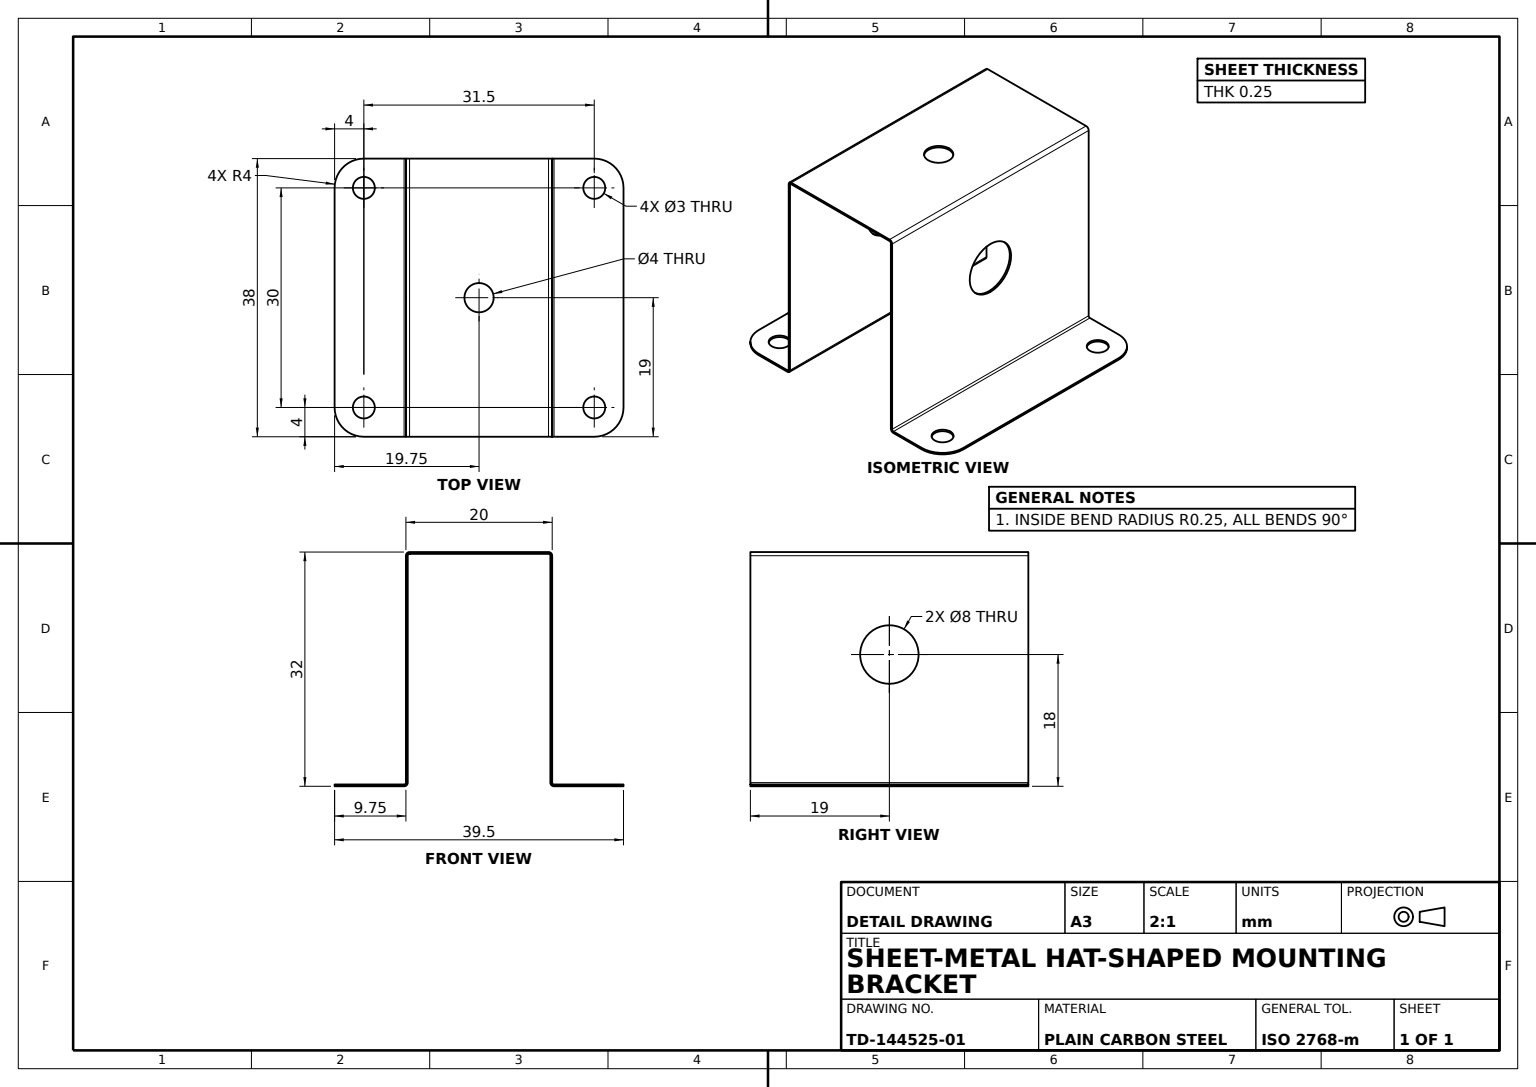
ISO-10303-21;
HEADER;
FILE_DESCRIPTION((''),'2;1');
FILE_NAME('','',(''),(''),'','','');
FILE_SCHEMA(('AUTOMOTIVE_DESIGN'));
ENDSEC;
DATA;
#1=APPLICATION_CONTEXT('');
#2=PRODUCT_CONTEXT('',#1,'mechanical');
#3=PRODUCT('','','',(#2));
#4=PRODUCT_DEFINITION_FORMATION('','',#3);
#5=PRODUCT_DEFINITION_CONTEXT('',#1,'design');
#6=PRODUCT_DEFINITION('','',#4,#5);
#7=PRODUCT_DEFINITION_SHAPE('','',#6);
#8=(LENGTH_UNIT()NAMED_UNIT(*)SI_UNIT(.MILLI.,.METRE.));
#9=(NAMED_UNIT(*)PLANE_ANGLE_UNIT()SI_UNIT($,.RADIAN.));
#10=(NAMED_UNIT(*)SI_UNIT($,.STERADIAN.)SOLID_ANGLE_UNIT());
#11=UNCERTAINTY_MEASURE_WITH_UNIT(LENGTH_MEASURE(1.E-05),#8,'distance_accuracy_value','');
#12=(GEOMETRIC_REPRESENTATION_CONTEXT(3)GLOBAL_UNCERTAINTY_ASSIGNED_CONTEXT((#11))GLOBAL_UNIT_ASSIGNED_CONTEXT((#8,#9,#10))REPRESENTATION_CONTEXT('',''));
#13=CARTESIAN_POINT('',(-10.25,-31.75,-19.));
#14=VERTEX_POINT('',#13);
#15=CARTESIAN_POINT('',(-10.25,-32.,-19.));
#16=VERTEX_POINT('',#15);
#17=DIRECTION('',(0.,-1.,0.));
#18=VECTOR('',#17,1000.);
#19=LINE('',#15,#18);
#20=EDGE_CURVE('',#14,#16,#19,.T.);
#21=ORIENTED_EDGE('',*,*,#20,.T.);
#22=CARTESIAN_POINT('',(-15.75,-32.,-19.));
#23=VERTEX_POINT('',#22);
#24=CARTESIAN_POINT('',(0.,-32.,-19.));
#25=DIRECTION('',(1.,0.,0.));
#26=VECTOR('',#25,1000.);
#27=LINE('',#24,#26);
#28=EDGE_CURVE('',#23,#16,#27,.T.);
#29=ORIENTED_EDGE('',*,*,#28,.F.);
#30=CARTESIAN_POINT('',(-15.75,-31.75,-19.));
#31=VERTEX_POINT('',#30);
#32=DIRECTION('',(0.,1.,0.));
#33=VECTOR('',#32,1000.);
#34=LINE('',#22,#33);
#35=EDGE_CURVE('',#23,#31,#34,.T.);
#36=ORIENTED_EDGE('',*,*,#35,.T.);
#37=CARTESIAN_POINT('',(-10.,-31.75,-19.));
#38=LINE('',#37,#26);
#39=EDGE_CURVE('',#31,#14,#38,.T.);
#40=ORIENTED_EDGE('',*,*,#39,.T.);
#41=EDGE_LOOP('',(#21,#29,#36,#40));
#42=FACE_OUTER_BOUND('',#41,.T.);
#43=CARTESIAN_POINT('',(-10.,-32.,-19.));
#44=DIRECTION('',(0.,0.,1.));
#45=AXIS2_PLACEMENT_3D('',#43,#44,#25);
#46=PLANE('',#45);
#47=ADVANCED_FACE('',(#42),#46,.F.);
#48=CARTESIAN_POINT('',(9.75,-0.5,19.));
#49=VERTEX_POINT('',#48);
#50=CARTESIAN_POINT('',(9.5,-0.25,19.));
#51=VERTEX_POINT('',#50);
#52=CARTESIAN_POINT('',(9.5,-0.5,19.));
#53=AXIS2_PLACEMENT_3D('',#52,#44,#25);
#54=CIRCLE('',#53,0.25);
#55=EDGE_CURVE('',#49,#51,#54,.T.);
#56=ORIENTED_EDGE('',*,*,#55,.T.);
#57=CARTESIAN_POINT('',(9.5,-0.25,-19.));
#58=VERTEX_POINT('',#57);
#59=DIRECTION('',(0.,0.,-1.));
#60=VECTOR('',#59,1000.);
#61=LINE('',#50,#60);
#62=EDGE_CURVE('',#51,#58,#61,.T.);
#63=ORIENTED_EDGE('',*,*,#62,.T.);
#64=CARTESIAN_POINT('',(9.75,-0.5,-19.));
#65=VERTEX_POINT('',#64);
#66=CARTESIAN_POINT('',(9.5,-0.5,-19.));
#67=DIRECTION('',(-1.,0.,0.));
#68=AXIS2_PLACEMENT_3D('',#66,#59,#67);
#69=CIRCLE('',#68,0.25);
#70=EDGE_CURVE('',#58,#65,#69,.T.);
#71=ORIENTED_EDGE('',*,*,#70,.T.);
#72=VECTOR('',#44,1000.);
#73=LINE('',#64,#72);
#74=EDGE_CURVE('',#65,#49,#73,.T.);
#75=ORIENTED_EDGE('',*,*,#74,.T.);
#76=EDGE_LOOP('',(#56,#63,#71,#75));
#77=FACE_OUTER_BOUND('',#76,.T.);
#78=CARTESIAN_POINT('',(9.5,-0.5,-38.005387));
#79=AXIS2_PLACEMENT_3D('',#78,#44,#25);
#80=CYLINDRICAL_SURFACE('',#79,0.25);
#81=ADVANCED_FACE('',(#77),#80,.F.);
#82=CARTESIAN_POINT('',(-9.5,-0.25,19.));
#83=VERTEX_POINT('',#82);
#84=CARTESIAN_POINT('',(-9.75,-0.5,19.));
#85=VERTEX_POINT('',#84);
#86=CARTESIAN_POINT('',(-9.5,-0.5,19.));
#87=AXIS2_PLACEMENT_3D('',#86,#44,#25);
#88=CIRCLE('',#87,0.25);
#89=EDGE_CURVE('',#83,#85,#88,.T.);
#90=ORIENTED_EDGE('',*,*,#89,.F.);
#91=CARTESIAN_POINT('',(-9.5,0.,19.));
#92=VERTEX_POINT('',#91);
#93=LINE('',#82,#33);
#94=EDGE_CURVE('',#83,#92,#93,.T.);
#95=ORIENTED_EDGE('',*,*,#94,.T.);
#96=CARTESIAN_POINT('',(-10.,-0.5,19.));
#97=VERTEX_POINT('',#96);
#98=AXIS2_PLACEMENT_3D('',#86,#44,#67);
#99=CIRCLE('',#98,0.5);
#100=EDGE_CURVE('',#92,#97,#99,.T.);
#101=ORIENTED_EDGE('',*,*,#100,.T.);
#102=VECTOR('',#67,1000.);
#103=LINE('',#96,#102);
#104=EDGE_CURVE('',#85,#97,#103,.T.);
#105=ORIENTED_EDGE('',*,*,#104,.F.);
#106=EDGE_LOOP('',(#90,#95,#101,#105));
#107=FACE_OUTER_BOUND('',#106,.T.);
#108=AXIS2_PLACEMENT_3D('',#86,#59,#67);
#109=PLANE('',#108);
#110=ADVANCED_FACE('',(#107),#109,.F.);
#111=CARTESIAN_POINT('',(-9.75,-18.,0.));
#112=VERTEX_POINT('',#111);
#113=CARTESIAN_POINT('',(-9.75,-10.,0.));
#114=VERTEX_POINT('',#113);
#115=CARTESIAN_POINT('',(-9.75,-14.,0.));
#116=AXIS2_PLACEMENT_3D('',#115,#67,#17);
#117=CIRCLE('',#116,4.);
#118=EDGE_CURVE('',#112,#114,#117,.T.);
#119=ORIENTED_EDGE('',*,*,#118,.F.);
#120=CARTESIAN_POINT('',(-10.,-18.,0.));
#121=VERTEX_POINT('',#120);
#122=CARTESIAN_POINT('',(19.75,-18.,0.));
#123=LINE('',#122,#102);
#124=EDGE_CURVE('',#112,#121,#123,.T.);
#125=ORIENTED_EDGE('',*,*,#124,.T.);
#126=CARTESIAN_POINT('',(-10.,-10.,0.));
#127=VERTEX_POINT('',#126);
#128=CARTESIAN_POINT('',(-10.,-14.,0.));
#129=AXIS2_PLACEMENT_3D('',#128,#67,#17);
#130=CIRCLE('',#129,4.);
#131=EDGE_CURVE('',#121,#127,#130,.T.);
#132=ORIENTED_EDGE('',*,*,#131,.T.);
#133=CARTESIAN_POINT('',(19.75,-10.,0.));
#134=LINE('',#133,#102);
#135=EDGE_CURVE('',#114,#127,#134,.T.);
#136=ORIENTED_EDGE('',*,*,#135,.F.);
#137=EDGE_LOOP('',(#119,#125,#132,#136));
#138=FACE_OUTER_BOUND('',#137,.T.);
#139=CARTESIAN_POINT('',(19.75,-14.,0.));
#140=AXIS2_PLACEMENT_3D('',#139,#67,#17);
#141=CYLINDRICAL_SURFACE('',#140,4.);
#142=ADVANCED_FACE('',(#138),#141,.F.);
#143=CARTESIAN_POINT('',(10.,-10.,0.));
#144=VERTEX_POINT('',#143);
#145=CARTESIAN_POINT('',(10.,-18.,0.));
#146=VERTEX_POINT('',#145);
#147=CARTESIAN_POINT('',(10.,-14.,0.));
#148=AXIS2_PLACEMENT_3D('',#147,#25,#32);
#149=CIRCLE('',#148,4.);
#150=EDGE_CURVE('',#144,#146,#149,.T.);
#151=ORIENTED_EDGE('',*,*,#150,.T.);
#152=CARTESIAN_POINT('',(9.75,-18.,0.));
#153=VERTEX_POINT('',#152);
#154=EDGE_CURVE('',#146,#153,#123,.T.);
#155=ORIENTED_EDGE('',*,*,#154,.T.);
#156=CARTESIAN_POINT('',(9.75,-10.,0.));
#157=VERTEX_POINT('',#156);
#158=CARTESIAN_POINT('',(9.75,-14.,0.));
#159=AXIS2_PLACEMENT_3D('',#158,#25,#32);
#160=CIRCLE('',#159,4.);
#161=EDGE_CURVE('',#157,#153,#160,.T.);
#162=ORIENTED_EDGE('',*,*,#161,.F.);
#163=EDGE_CURVE('',#144,#157,#134,.T.);
#164=ORIENTED_EDGE('',*,*,#163,.F.);
#165=EDGE_LOOP('',(#151,#155,#162,#164));
#166=FACE_OUTER_BOUND('',#165,.T.);
#167=ADVANCED_FACE('',(#166),#141,.F.);
#168=CARTESIAN_POINT('',(-9.75,-0.5,-19.));
#169=VERTEX_POINT('',#168);
#170=CARTESIAN_POINT('',(-10.,-0.5,-19.));
#171=VERTEX_POINT('',#170);
#172=LINE('',#168,#102);
#173=EDGE_CURVE('',#169,#171,#172,.T.);
#174=ORIENTED_EDGE('',*,*,#173,.T.);
#175=CARTESIAN_POINT('',(-9.5,0.,-19.));
#176=VERTEX_POINT('',#175);
#177=CARTESIAN_POINT('',(-9.5,-0.5,-19.));
#178=AXIS2_PLACEMENT_3D('',#177,#59,#67);
#179=CIRCLE('',#178,0.5);
#180=EDGE_CURVE('',#171,#176,#179,.T.);
#181=ORIENTED_EDGE('',*,*,#180,.T.);
#182=CARTESIAN_POINT('',(-9.5,-0.25,-19.));
#183=VERTEX_POINT('',#182);
#184=LINE('',#182,#33);
#185=EDGE_CURVE('',#183,#176,#184,.T.);
#186=ORIENTED_EDGE('',*,*,#185,.F.);
#187=CIRCLE('',#178,0.25);
#188=EDGE_CURVE('',#169,#183,#187,.T.);
#189=ORIENTED_EDGE('',*,*,#188,.F.);
#190=EDGE_LOOP('',(#174,#181,#186,#189));
#191=FACE_OUTER_BOUND('',#190,.T.);
#192=AXIS2_PLACEMENT_3D('',#177,#44,#25);
#193=PLANE('',#192);
#194=ADVANCED_FACE('',(#191),#193,.F.);
#195=CARTESIAN_POINT('',(-15.75,-31.75,19.));
#196=VERTEX_POINT('',#195);
#197=CARTESIAN_POINT('',(-15.75,-32.,19.));
#198=VERTEX_POINT('',#197);
#199=LINE('',#197,#18);
#200=EDGE_CURVE('',#196,#198,#199,.T.);
#201=ORIENTED_EDGE('',*,*,#200,.F.);
#202=CARTESIAN_POINT('',(-19.75,-31.75,15.));
#203=VERTEX_POINT('',#202);
#204=CARTESIAN_POINT('',(-15.75,-31.75,15.));
#205=AXIS2_PLACEMENT_3D('',#204,#32,#44);
#206=CIRCLE('',#205,4.);
#207=EDGE_CURVE('',#203,#196,#206,.T.);
#208=ORIENTED_EDGE('',*,*,#207,.F.);
#209=CARTESIAN_POINT('',(-19.75,-32.,15.));
#210=VERTEX_POINT('',#209);
#211=LINE('',#209,#33);
#212=EDGE_CURVE('',#210,#203,#211,.T.);
#213=ORIENTED_EDGE('',*,*,#212,.F.);
#214=CARTESIAN_POINT('',(-15.75,-32.,15.));
#215=AXIS2_PLACEMENT_3D('',#214,#17,#44);
#216=CIRCLE('',#215,4.);
#217=EDGE_CURVE('',#198,#210,#216,.T.);
#218=ORIENTED_EDGE('',*,*,#217,.F.);
#219=EDGE_LOOP('',(#201,#208,#213,#218));
#220=FACE_OUTER_BOUND('',#219,.T.);
#221=AXIS2_PLACEMENT_3D('',#214,#32,#67);
#222=CYLINDRICAL_SURFACE('',#221,4.);
#223=ADVANCED_FACE('',(#220),#222,.T.);
#224=CARTESIAN_POINT('',(10.25,-32.,-19.));
#225=VERTEX_POINT('',#224);
#226=CARTESIAN_POINT('',(15.75,-32.,-19.));
#227=VERTEX_POINT('',#226);
#228=EDGE_CURVE('',#225,#227,#27,.T.);
#229=ORIENTED_EDGE('',*,*,#228,.F.);
#230=CARTESIAN_POINT('',(10.25,-31.75,-19.));
#231=VERTEX_POINT('',#230);
#232=LINE('',#230,#18);
#233=EDGE_CURVE('',#231,#225,#232,.T.);
#234=ORIENTED_EDGE('',*,*,#233,.F.);
#235=CARTESIAN_POINT('',(15.75,-31.75,-19.));
#236=VERTEX_POINT('',#235);
#237=CARTESIAN_POINT('',(19.75,-31.75,-19.));
#238=LINE('',#237,#26);
#239=EDGE_CURVE('',#231,#236,#238,.T.);
#240=ORIENTED_EDGE('',*,*,#239,.T.);
#241=LINE('',#226,#18);
#242=EDGE_CURVE('',#236,#227,#241,.T.);
#243=ORIENTED_EDGE('',*,*,#242,.T.);
#244=EDGE_LOOP('',(#229,#234,#240,#243));
#245=FACE_OUTER_BOUND('',#244,.T.);
#246=CARTESIAN_POINT('',(19.75,-32.,-19.));
#247=AXIS2_PLACEMENT_3D('',#246,#44,#25);
#248=PLANE('',#247);
#249=ADVANCED_FACE('',(#245),#248,.F.);
#250=CARTESIAN_POINT('',(9.75,-31.5,-19.));
#251=VERTEX_POINT('',#250);
#252=CARTESIAN_POINT('',(10.25,-31.5,-19.));
#253=AXIS2_PLACEMENT_3D('',#252,#44,#17);
#254=CIRCLE('',#253,0.5);
#255=EDGE_CURVE('',#251,#225,#254,.T.);
#256=ORIENTED_EDGE('',*,*,#255,.F.);
#257=CARTESIAN_POINT('',(10.,-31.5,-19.));
#258=VERTEX_POINT('',#257);
#259=LINE('',#257,#102);
#260=EDGE_CURVE('',#258,#251,#259,.T.);
#261=ORIENTED_EDGE('',*,*,#260,.F.);
#262=CIRCLE('',#253,0.25);
#263=EDGE_CURVE('',#258,#231,#262,.T.);
#264=ORIENTED_EDGE('',*,*,#263,.T.);
#265=ORIENTED_EDGE('',*,*,#233,.T.);
#266=EDGE_LOOP('',(#256,#261,#264,#265));
#267=FACE_OUTER_BOUND('',#266,.T.);
#268=AXIS2_PLACEMENT_3D('',#252,#59,#32);
#269=PLANE('',#268);
#270=ADVANCED_FACE('',(#267),#269,.T.);
#271=LINE('',#175,#72);
#272=EDGE_CURVE('',#176,#92,#271,.T.);
#273=ORIENTED_EDGE('',*,*,#272,.F.);
#274=ORIENTED_EDGE('',*,*,#180,.F.);
#275=CARTESIAN_POINT('',(-10.,-0.5,0.));
#276=LINE('',#275,#60);
#277=EDGE_CURVE('',#97,#171,#276,.T.);
#278=ORIENTED_EDGE('',*,*,#277,.F.);
#279=ORIENTED_EDGE('',*,*,#100,.F.);
#280=EDGE_LOOP('',(#273,#274,#278,#279));
#281=FACE_OUTER_BOUND('',#280,.T.);
#282=CARTESIAN_POINT('',(-9.5,-0.5,38.005387));
#283=AXIS2_PLACEMENT_3D('',#282,#59,#67);
#284=CYLINDRICAL_SURFACE('',#283,0.5);
#285=ADVANCED_FACE('',(#281),#284,.T.);
#286=CARTESIAN_POINT('',(-9.75,-31.5,-19.));
#287=VERTEX_POINT('',#286);
#288=CARTESIAN_POINT('',(-10.25,-31.5,-19.));
#289=AXIS2_PLACEMENT_3D('',#288,#44,#32);
#290=CIRCLE('',#289,0.5);
#291=EDGE_CURVE('',#16,#287,#290,.T.);
#292=ORIENTED_EDGE('',*,*,#291,.T.);
#293=CARTESIAN_POINT('',(-9.75,-31.5,19.));
#294=VERTEX_POINT('',#293);
#295=LINE('',#293,#60);
#296=EDGE_CURVE('',#294,#287,#295,.T.);
#297=ORIENTED_EDGE('',*,*,#296,.F.);
#298=CARTESIAN_POINT('',(-10.25,-32.,19.));
#299=VERTEX_POINT('',#298);
#300=CARTESIAN_POINT('',(-10.25,-31.5,19.));
#301=AXIS2_PLACEMENT_3D('',#300,#59,#17);
#302=CIRCLE('',#301,0.5);
#303=EDGE_CURVE('',#294,#299,#302,.T.);
#304=ORIENTED_EDGE('',*,*,#303,.T.);
#305=LINE('',#15,#60);
#306=EDGE_CURVE('',#299,#16,#305,.T.);
#307=ORIENTED_EDGE('',*,*,#306,.T.);
#308=EDGE_LOOP('',(#292,#297,#304,#307));
#309=FACE_OUTER_BOUND('',#308,.T.);
#310=CARTESIAN_POINT('',(-10.25,-31.5,38.005387));
#311=AXIS2_PLACEMENT_3D('',#310,#59,#17);
#312=CYLINDRICAL_SURFACE('',#311,0.5);
#313=ADVANCED_FACE('',(#309),#312,.T.);
#314=CARTESIAN_POINT('',(10.,-31.5,19.));
#315=VERTEX_POINT('',#314);
#316=CARTESIAN_POINT('',(9.75,-31.5,19.));
#317=VERTEX_POINT('',#316);
#318=LINE('',#314,#102);
#319=EDGE_CURVE('',#315,#317,#318,.T.);
#320=ORIENTED_EDGE('',*,*,#319,.T.);
#321=CARTESIAN_POINT('',(10.25,-32.,19.));
#322=VERTEX_POINT('',#321);
#323=CARTESIAN_POINT('',(10.25,-31.5,19.));
#324=AXIS2_PLACEMENT_3D('',#323,#59,#32);
#325=CIRCLE('',#324,0.5);
#326=EDGE_CURVE('',#322,#317,#325,.T.);
#327=ORIENTED_EDGE('',*,*,#326,.F.);
#328=CARTESIAN_POINT('',(10.25,-31.75,19.));
#329=VERTEX_POINT('',#328);
#330=LINE('',#321,#18);
#331=EDGE_CURVE('',#329,#322,#330,.T.);
#332=ORIENTED_EDGE('',*,*,#331,.F.);
#333=AXIS2_PLACEMENT_3D('',#323,#59,#17);
#334=CIRCLE('',#333,0.25);
#335=EDGE_CURVE('',#329,#315,#334,.T.);
#336=ORIENTED_EDGE('',*,*,#335,.T.);
#337=EDGE_LOOP('',(#320,#327,#332,#336));
#338=FACE_OUTER_BOUND('',#337,.T.);
#339=AXIS2_PLACEMENT_3D('',#323,#44,#17);
#340=PLANE('',#339);
#341=ADVANCED_FACE('',(#338),#340,.T.);
#342=ORIENTED_EDGE('',*,*,#331,.T.);
#343=CARTESIAN_POINT('',(15.75,-32.,19.));
#344=VERTEX_POINT('',#343);
#345=CARTESIAN_POINT('',(0.,-32.,19.));
#346=LINE('',#345,#102);
#347=EDGE_CURVE('',#344,#322,#346,.T.);
#348=ORIENTED_EDGE('',*,*,#347,.F.);
#349=CARTESIAN_POINT('',(15.75,-31.75,19.));
#350=VERTEX_POINT('',#349);
#351=LINE('',#343,#33);
#352=EDGE_CURVE('',#344,#350,#351,.T.);
#353=ORIENTED_EDGE('',*,*,#352,.T.);
#354=CARTESIAN_POINT('',(10.,-31.75,19.));
#355=LINE('',#354,#102);
#356=EDGE_CURVE('',#350,#329,#355,.T.);
#357=ORIENTED_EDGE('',*,*,#356,.T.);
#358=EDGE_LOOP('',(#342,#348,#353,#357));
#359=FACE_OUTER_BOUND('',#358,.T.);
#360=CARTESIAN_POINT('',(10.,-32.,19.));
#361=AXIS2_PLACEMENT_3D('',#360,#59,#67);
#362=PLANE('',#361);
#363=ADVANCED_FACE('',(#359),#362,.F.);
#364=ORIENTED_EDGE('',*,*,#291,.F.);
#365=ORIENTED_EDGE('',*,*,#20,.F.);
#366=CARTESIAN_POINT('',(-10.,-31.5,-19.));
#367=VERTEX_POINT('',#366);
#368=AXIS2_PLACEMENT_3D('',#288,#44,#17);
#369=CIRCLE('',#368,0.25);
#370=EDGE_CURVE('',#14,#367,#369,.T.);
#371=ORIENTED_EDGE('',*,*,#370,.T.);
#372=LINE('',#366,#26);
#373=EDGE_CURVE('',#367,#287,#372,.T.);
#374=ORIENTED_EDGE('',*,*,#373,.T.);
#375=EDGE_LOOP('',(#364,#365,#371,#374));
#376=FACE_OUTER_BOUND('',#375,.T.);
#377=AXIS2_PLACEMENT_3D('',#288,#59,#17);
#378=PLANE('',#377);
#379=ADVANCED_FACE('',(#376),#378,.T.);
#380=CARTESIAN_POINT('',(15.75,-32.,-13.5));
#381=VERTEX_POINT('',#380);
#382=CARTESIAN_POINT('',(15.75,-31.75,-13.5));
#383=VERTEX_POINT('',#382);
#384=CARTESIAN_POINT('',(15.75,-41.75,-13.5));
#385=LINE('',#384,#33);
#386=EDGE_CURVE('',#381,#383,#385,.T.);
#387=ORIENTED_EDGE('',*,*,#386,.T.);
#388=CARTESIAN_POINT('',(15.75,-31.75,-16.5));
#389=VERTEX_POINT('',#388);
#390=CARTESIAN_POINT('',(15.75,-31.75,-15.));
#391=AXIS2_PLACEMENT_3D('',#390,#32,#44);
#392=CIRCLE('',#391,1.5);
#393=EDGE_CURVE('',#383,#389,#392,.T.);
#394=ORIENTED_EDGE('',*,*,#393,.T.);
#395=CARTESIAN_POINT('',(15.75,-32.,-16.5));
#396=VERTEX_POINT('',#395);
#397=CARTESIAN_POINT('',(15.75,-41.75,-16.5));
#398=LINE('',#397,#33);
#399=EDGE_CURVE('',#396,#389,#398,.T.);
#400=ORIENTED_EDGE('',*,*,#399,.F.);
#401=CARTESIAN_POINT('',(15.75,-32.,-15.));
#402=AXIS2_PLACEMENT_3D('',#401,#32,#44);
#403=CIRCLE('',#402,1.5);
#404=EDGE_CURVE('',#381,#396,#403,.T.);
#405=ORIENTED_EDGE('',*,*,#404,.F.);
#406=EDGE_LOOP('',(#387,#394,#400,#405));
#407=FACE_OUTER_BOUND('',#406,.T.);
#408=CARTESIAN_POINT('',(15.75,-41.75,-15.));
#409=AXIS2_PLACEMENT_3D('',#408,#32,#44);
#410=CYLINDRICAL_SURFACE('',#409,1.5);
#411=ADVANCED_FACE('',(#407),#410,.F.);
#412=CARTESIAN_POINT('',(-15.75,-32.,13.5));
#413=VERTEX_POINT('',#412);
#414=CARTESIAN_POINT('',(-15.75,-32.,16.5));
#415=VERTEX_POINT('',#414);
#416=AXIS2_PLACEMENT_3D('',#214,#32,#44);
#417=CIRCLE('',#416,1.5);
#418=EDGE_CURVE('',#413,#415,#417,.T.);
#419=ORIENTED_EDGE('',*,*,#418,.T.);
#420=EDGE_CURVE('',#415,#413,#417,.T.);
#421=ORIENTED_EDGE('',*,*,#420,.T.);
#422=EDGE_LOOP('',(#419,#421));
#423=FACE_BOUND('',#422,.T.);
#424=ORIENTED_EDGE('',*,*,#28,.T.);
#425=ORIENTED_EDGE('',*,*,#306,.F.);
#426=EDGE_CURVE('',#299,#198,#346,.T.);
#427=ORIENTED_EDGE('',*,*,#426,.T.);
#428=ORIENTED_EDGE('',*,*,#217,.T.);
#429=CARTESIAN_POINT('',(-19.75,-32.,-15.));
#430=VERTEX_POINT('',#429);
#431=CARTESIAN_POINT('',(-19.75,-32.,0.));
#432=LINE('',#431,#60);
#433=EDGE_CURVE('',#210,#430,#432,.T.);
#434=ORIENTED_EDGE('',*,*,#433,.T.);
#435=CARTESIAN_POINT('',(-15.75,-32.,-15.));
#436=AXIS2_PLACEMENT_3D('',#435,#17,#44);
#437=CIRCLE('',#436,4.);
#438=EDGE_CURVE('',#430,#23,#437,.T.);
#439=ORIENTED_EDGE('',*,*,#438,.T.);
#440=EDGE_LOOP('',(#424,#425,#427,#428,#434,#439));
#441=FACE_OUTER_BOUND('',#440,.T.);
#442=CARTESIAN_POINT('',(-15.75,-32.,-13.5));
#443=VERTEX_POINT('',#442);
#444=CARTESIAN_POINT('',(-15.75,-32.,-16.5));
#445=VERTEX_POINT('',#444);
#446=AXIS2_PLACEMENT_3D('',#435,#32,#44);
#447=CIRCLE('',#446,1.5);
#448=EDGE_CURVE('',#443,#445,#447,.T.);
#449=ORIENTED_EDGE('',*,*,#448,.T.);
#450=EDGE_CURVE('',#445,#443,#447,.T.);
#451=ORIENTED_EDGE('',*,*,#450,.T.);
#452=EDGE_LOOP('',(#449,#451));
#453=FACE_BOUND('',#452,.T.);
#454=CARTESIAN_POINT('',(0.,-32.,0.));
#455=AXIS2_PLACEMENT_3D('',#454,#32,#44);
#456=PLANE('',#455);
#457=ADVANCED_FACE('',(#423,#441,#453),#456,.F.);
#458=CARTESIAN_POINT('',(-15.75,-31.75,-13.5));
#459=VERTEX_POINT('',#458);
#460=CARTESIAN_POINT('',(-15.75,-31.75,-16.5));
#461=VERTEX_POINT('',#460);
#462=CARTESIAN_POINT('',(-15.75,-31.75,-15.));
#463=AXIS2_PLACEMENT_3D('',#462,#32,#44);
#464=CIRCLE('',#463,1.5);
#465=EDGE_CURVE('',#459,#461,#464,.T.);
#466=ORIENTED_EDGE('',*,*,#465,.T.);
#467=CARTESIAN_POINT('',(-15.75,-41.75,-16.5));
#468=LINE('',#467,#33);
#469=EDGE_CURVE('',#445,#461,#468,.T.);
#470=ORIENTED_EDGE('',*,*,#469,.F.);
#471=ORIENTED_EDGE('',*,*,#448,.F.);
#472=CARTESIAN_POINT('',(-15.75,-41.75,-13.5));
#473=LINE('',#472,#33);
#474=EDGE_CURVE('',#443,#459,#473,.T.);
#475=ORIENTED_EDGE('',*,*,#474,.T.);
#476=EDGE_LOOP('',(#466,#470,#471,#475));
#477=FACE_OUTER_BOUND('',#476,.T.);
#478=CARTESIAN_POINT('',(-15.75,-41.75,-15.));
#479=AXIS2_PLACEMENT_3D('',#478,#32,#44);
#480=CYLINDRICAL_SURFACE('',#479,1.5);
#481=ADVANCED_FACE('',(#477),#480,.F.);
#482=CARTESIAN_POINT('',(10.,-0.5,-19.));
#483=VERTEX_POINT('',#482);
#484=CARTESIAN_POINT('',(10.,-0.5,19.));
#485=VERTEX_POINT('',#484);
#486=CARTESIAN_POINT('',(10.,-0.5,0.));
#487=LINE('',#486,#72);
#488=EDGE_CURVE('',#483,#485,#487,.T.);
#489=ORIENTED_EDGE('',*,*,#488,.F.);
#490=CARTESIAN_POINT('',(9.5,0.,-19.));
#491=VERTEX_POINT('',#490);
#492=AXIS2_PLACEMENT_3D('',#66,#59,#25);
#493=CIRCLE('',#492,0.5);
#494=EDGE_CURVE('',#491,#483,#493,.T.);
#495=ORIENTED_EDGE('',*,*,#494,.F.);
#496=CARTESIAN_POINT('',(9.5,0.,19.));
#497=VERTEX_POINT('',#496);
#498=LINE('',#496,#60);
#499=EDGE_CURVE('',#497,#491,#498,.T.);
#500=ORIENTED_EDGE('',*,*,#499,.F.);
#501=CIRCLE('',#53,0.5);
#502=EDGE_CURVE('',#485,#497,#501,.T.);
#503=ORIENTED_EDGE('',*,*,#502,.F.);
#504=EDGE_LOOP('',(#489,#495,#500,#503));
#505=FACE_OUTER_BOUND('',#504,.T.);
#506=CYLINDRICAL_SURFACE('',#79,0.5);
#507=ADVANCED_FACE('',(#505),#506,.T.);
#508=EDGE_CURVE('',#114,#112,#117,.T.);
#509=ORIENTED_EDGE('',*,*,#508,.T.);
#510=ORIENTED_EDGE('',*,*,#118,.T.);
#511=EDGE_LOOP('',(#509,#510));
#512=FACE_BOUND('',#511,.T.);
#513=LINE('',#84,#60);
#514=EDGE_CURVE('',#85,#169,#513,.T.);
#515=ORIENTED_EDGE('',*,*,#514,.F.);
#516=CARTESIAN_POINT('',(-9.75,0.,19.));
#517=LINE('',#516,#18);
#518=EDGE_CURVE('',#85,#294,#517,.T.);
#519=ORIENTED_EDGE('',*,*,#518,.T.);
#520=ORIENTED_EDGE('',*,*,#296,.T.);
#521=CARTESIAN_POINT('',(-9.75,0.,-19.));
#522=LINE('',#521,#33);
#523=EDGE_CURVE('',#287,#169,#522,.T.);
#524=ORIENTED_EDGE('',*,*,#523,.T.);
#525=EDGE_LOOP('',(#515,#519,#520,#524));
#526=FACE_OUTER_BOUND('',#525,.T.);
#527=CARTESIAN_POINT('',(-9.75,0.,0.));
#528=AXIS2_PLACEMENT_3D('',#527,#67,#17);
#529=PLANE('',#528);
#530=ADVANCED_FACE('',(#512,#526),#529,.F.);
#531=CARTESIAN_POINT('',(15.75,-32.,13.5));
#532=VERTEX_POINT('',#531);
#533=CARTESIAN_POINT('',(15.75,-31.75,13.5));
#534=VERTEX_POINT('',#533);
#535=CARTESIAN_POINT('',(15.75,-41.75,13.5));
#536=LINE('',#535,#33);
#537=EDGE_CURVE('',#532,#534,#536,.T.);
#538=ORIENTED_EDGE('',*,*,#537,.T.);
#539=CARTESIAN_POINT('',(15.75,-31.75,16.5));
#540=VERTEX_POINT('',#539);
#541=CARTESIAN_POINT('',(15.75,-31.75,15.));
#542=AXIS2_PLACEMENT_3D('',#541,#32,#44);
#543=CIRCLE('',#542,1.5);
#544=EDGE_CURVE('',#534,#540,#543,.T.);
#545=ORIENTED_EDGE('',*,*,#544,.T.);
#546=CARTESIAN_POINT('',(15.75,-32.,16.5));
#547=VERTEX_POINT('',#546);
#548=CARTESIAN_POINT('',(15.75,-41.75,16.5));
#549=LINE('',#548,#33);
#550=EDGE_CURVE('',#547,#540,#549,.T.);
#551=ORIENTED_EDGE('',*,*,#550,.F.);
#552=CARTESIAN_POINT('',(15.75,-32.,15.));
#553=AXIS2_PLACEMENT_3D('',#552,#32,#44);
#554=CIRCLE('',#553,1.5);
#555=EDGE_CURVE('',#532,#547,#554,.T.);
#556=ORIENTED_EDGE('',*,*,#555,.F.);
#557=EDGE_LOOP('',(#538,#545,#551,#556));
#558=FACE_OUTER_BOUND('',#557,.T.);
#559=CARTESIAN_POINT('',(15.75,-41.75,15.));
#560=AXIS2_PLACEMENT_3D('',#559,#32,#44);
#561=CYLINDRICAL_SURFACE('',#560,1.5);
#562=ADVANCED_FACE('',(#558),#561,.F.);
#563=ORIENTED_EDGE('',*,*,#272,.T.);
#564=CARTESIAN_POINT('',(-10.,0.,19.));
#565=LINE('',#564,#26);
#566=EDGE_CURVE('',#92,#497,#565,.T.);
#567=ORIENTED_EDGE('',*,*,#566,.T.);
#568=ORIENTED_EDGE('',*,*,#499,.T.);
#569=CARTESIAN_POINT('',(-10.,0.,-19.));
#570=LINE('',#569,#102);
#571=EDGE_CURVE('',#491,#176,#570,.T.);
#572=ORIENTED_EDGE('',*,*,#571,.T.);
#573=EDGE_LOOP('',(#563,#567,#568,#572));
#574=FACE_OUTER_BOUND('',#573,.T.);
#575=CARTESIAN_POINT('',(0.,0.,2.));
#576=VERTEX_POINT('',#575);
#577=CARTESIAN_POINT('',(0.,0.,-2.));
#578=VERTEX_POINT('',#577);
#579=CARTESIAN_POINT('',(0.,0.,0.));
#580=AXIS2_PLACEMENT_3D('',#579,#32,#44);
#581=CIRCLE('',#580,2.);
#582=EDGE_CURVE('',#576,#578,#581,.T.);
#583=ORIENTED_EDGE('',*,*,#582,.F.);
#584=EDGE_CURVE('',#578,#576,#581,.T.);
#585=ORIENTED_EDGE('',*,*,#584,.F.);
#586=EDGE_LOOP('',(#583,#585));
#587=FACE_BOUND('',#586,.T.);
#588=PLANE('',#580);
#589=ADVANCED_FACE('',(#574,#587),#588,.T.);
#590=CARTESIAN_POINT('',(-10.,-31.5,19.));
#591=VERTEX_POINT('',#590);
#592=CARTESIAN_POINT('',(-10.25,-31.75,19.));
#593=VERTEX_POINT('',#592);
#594=CIRCLE('',#301,0.25);
#595=EDGE_CURVE('',#591,#593,#594,.T.);
#596=ORIENTED_EDGE('',*,*,#595,.F.);
#597=LINE('',#590,#60);
#598=EDGE_CURVE('',#591,#367,#597,.T.);
#599=ORIENTED_EDGE('',*,*,#598,.T.);
#600=ORIENTED_EDGE('',*,*,#370,.F.);
#601=LINE('',#13,#72);
#602=EDGE_CURVE('',#14,#593,#601,.T.);
#603=ORIENTED_EDGE('',*,*,#602,.T.);
#604=EDGE_LOOP('',(#596,#599,#600,#603));
#605=FACE_OUTER_BOUND('',#604,.T.);
#606=CYLINDRICAL_SURFACE('',#311,0.25);
#607=ADVANCED_FACE('',(#605),#606,.F.);
#608=ORIENTED_EDGE('',*,*,#212,.T.);
#609=CARTESIAN_POINT('',(-19.75,-31.75,-15.));
#610=VERTEX_POINT('',#609);
#611=CARTESIAN_POINT('',(-19.75,-31.75,-19.));
#612=LINE('',#611,#60);
#613=EDGE_CURVE('',#203,#610,#612,.T.);
#614=ORIENTED_EDGE('',*,*,#613,.T.);
#615=LINE('',#429,#18);
#616=EDGE_CURVE('',#610,#430,#615,.T.);
#617=ORIENTED_EDGE('',*,*,#616,.T.);
#618=ORIENTED_EDGE('',*,*,#433,.F.);
#619=EDGE_LOOP('',(#608,#614,#617,#618));
#620=FACE_OUTER_BOUND('',#619,.T.);
#621=CARTESIAN_POINT('',(-19.75,-32.,-19.));
#622=AXIS2_PLACEMENT_3D('',#621,#25,#32);
#623=PLANE('',#622);
#624=ADVANCED_FACE('',(#620),#623,.F.);
#625=LINE('',#57,#33);
#626=EDGE_CURVE('',#58,#491,#625,.T.);
#627=ORIENTED_EDGE('',*,*,#626,.F.);
#628=CARTESIAN_POINT('',(-10.,-0.25,-19.));
#629=LINE('',#628,#102);
#630=EDGE_CURVE('',#58,#183,#629,.T.);
#631=ORIENTED_EDGE('',*,*,#630,.T.);
#632=ORIENTED_EDGE('',*,*,#185,.T.);
#633=ORIENTED_EDGE('',*,*,#571,.F.);
#634=EDGE_LOOP('',(#627,#631,#632,#633));
#635=FACE_OUTER_BOUND('',#634,.T.);
#636=AXIS2_PLACEMENT_3D('',#628,#59,#67);
#637=PLANE('',#636);
#638=ADVANCED_FACE('',(#635),#637,.T.);
#639=EDGE_CURVE('',#540,#534,#543,.T.);
#640=ORIENTED_EDGE('',*,*,#639,.T.);
#641=ORIENTED_EDGE('',*,*,#537,.F.);
#642=EDGE_CURVE('',#547,#532,#554,.T.);
#643=ORIENTED_EDGE('',*,*,#642,.F.);
#644=ORIENTED_EDGE('',*,*,#550,.T.);
#645=EDGE_LOOP('',(#640,#641,#643,#644));
#646=FACE_OUTER_BOUND('',#645,.T.);
#647=ADVANCED_FACE('',(#646),#561,.F.);
#648=ORIENTED_EDGE('',*,*,#263,.F.);
#649=LINE('',#257,#72);
#650=EDGE_CURVE('',#258,#315,#649,.T.);
#651=ORIENTED_EDGE('',*,*,#650,.T.);
#652=ORIENTED_EDGE('',*,*,#335,.F.);
#653=LINE('',#328,#60);
#654=EDGE_CURVE('',#329,#231,#653,.T.);
#655=ORIENTED_EDGE('',*,*,#654,.T.);
#656=EDGE_LOOP('',(#648,#651,#652,#655));
#657=FACE_OUTER_BOUND('',#656,.T.);
#658=CARTESIAN_POINT('',(10.25,-31.5,-38.005387));
#659=AXIS2_PLACEMENT_3D('',#658,#44,#17);
#660=CYLINDRICAL_SURFACE('',#659,0.25);
#661=ADVANCED_FACE('',(#657),#660,.F.);
#662=ORIENTED_EDGE('',*,*,#319,.F.);
#663=CARTESIAN_POINT('',(10.,-0.25,19.));
#664=LINE('',#663,#33);
#665=EDGE_CURVE('',#315,#485,#664,.T.);
#666=ORIENTED_EDGE('',*,*,#665,.T.);
#667=LINE('',#48,#26);
#668=EDGE_CURVE('',#49,#485,#667,.T.);
#669=ORIENTED_EDGE('',*,*,#668,.F.);
#670=CARTESIAN_POINT('',(9.75,0.,19.));
#671=LINE('',#670,#33);
#672=EDGE_CURVE('',#317,#49,#671,.T.);
#673=ORIENTED_EDGE('',*,*,#672,.F.);
#674=EDGE_LOOP('',(#662,#666,#669,#673));
#675=FACE_OUTER_BOUND('',#674,.T.);
#676=AXIS2_PLACEMENT_3D('',#663,#44,#17);
#677=PLANE('',#676);
#678=ADVANCED_FACE('',(#675),#677,.T.);
#679=ORIENTED_EDGE('',*,*,#523,.F.);
#680=ORIENTED_EDGE('',*,*,#373,.F.);
#681=LINE('',#628,#33);
#682=EDGE_CURVE('',#367,#171,#681,.T.);
#683=ORIENTED_EDGE('',*,*,#682,.T.);
#684=ORIENTED_EDGE('',*,*,#173,.F.);
#685=EDGE_LOOP('',(#679,#680,#683,#684));
#686=FACE_OUTER_BOUND('',#685,.T.);
#687=AXIS2_PLACEMENT_3D('',#628,#59,#32);
#688=PLANE('',#687);
#689=ADVANCED_FACE('',(#686),#688,.T.);
#690=CARTESIAN_POINT('',(19.75,-31.75,15.));
#691=VERTEX_POINT('',#690);
#692=CARTESIAN_POINT('',(19.75,-32.,15.));
#693=VERTEX_POINT('',#692);
#694=LINE('',#692,#18);
#695=EDGE_CURVE('',#691,#693,#694,.T.);
#696=ORIENTED_EDGE('',*,*,#695,.T.);
#697=CARTESIAN_POINT('',(19.75,-32.,-15.));
#698=VERTEX_POINT('',#697);
#699=CARTESIAN_POINT('',(19.75,-32.,0.));
#700=LINE('',#699,#72);
#701=EDGE_CURVE('',#698,#693,#700,.T.);
#702=ORIENTED_EDGE('',*,*,#701,.F.);
#703=CARTESIAN_POINT('',(19.75,-31.75,-15.));
#704=VERTEX_POINT('',#703);
#705=LINE('',#697,#33);
#706=EDGE_CURVE('',#698,#704,#705,.T.);
#707=ORIENTED_EDGE('',*,*,#706,.T.);
#708=CARTESIAN_POINT('',(19.75,-31.75,19.));
#709=LINE('',#708,#72);
#710=EDGE_CURVE('',#704,#691,#709,.T.);
#711=ORIENTED_EDGE('',*,*,#710,.T.);
#712=EDGE_LOOP('',(#696,#702,#707,#711));
#713=FACE_OUTER_BOUND('',#712,.T.);
#714=CARTESIAN_POINT('',(19.75,-32.,19.));
#715=AXIS2_PLACEMENT_3D('',#714,#67,#44);
#716=PLANE('',#715);
#717=ADVANCED_FACE('',(#713),#716,.F.);
#718=ORIENTED_EDGE('',*,*,#418,.F.);
#719=CARTESIAN_POINT('',(-15.75,-31.75,13.5));
#720=VERTEX_POINT('',#719);
#721=CARTESIAN_POINT('',(-15.75,-41.75,13.5));
#722=LINE('',#721,#33);
#723=EDGE_CURVE('',#413,#720,#722,.T.);
#724=ORIENTED_EDGE('',*,*,#723,.T.);
#725=CARTESIAN_POINT('',(-15.75,-31.75,16.5));
#726=VERTEX_POINT('',#725);
#727=CIRCLE('',#205,1.5);
#728=EDGE_CURVE('',#720,#726,#727,.T.);
#729=ORIENTED_EDGE('',*,*,#728,.T.);
#730=CARTESIAN_POINT('',(-15.75,-41.75,16.5));
#731=LINE('',#730,#33);
#732=EDGE_CURVE('',#415,#726,#731,.T.);
#733=ORIENTED_EDGE('',*,*,#732,.F.);
#734=EDGE_LOOP('',(#718,#724,#729,#733));
#735=FACE_OUTER_BOUND('',#734,.T.);
#736=CARTESIAN_POINT('',(-15.75,-41.75,15.));
#737=AXIS2_PLACEMENT_3D('',#736,#32,#44);
#738=CYLINDRICAL_SURFACE('',#737,1.5);
#739=ADVANCED_FACE('',(#735),#738,.F.);
#740=ORIENTED_EDGE('',*,*,#94,.F.);
#741=CARTESIAN_POINT('',(-10.,-0.25,19.));
#742=LINE('',#741,#26);
#743=EDGE_CURVE('',#83,#51,#742,.T.);
#744=ORIENTED_EDGE('',*,*,#743,.T.);
#745=LINE('',#50,#33);
#746=EDGE_CURVE('',#51,#497,#745,.T.);
#747=ORIENTED_EDGE('',*,*,#746,.T.);
#748=ORIENTED_EDGE('',*,*,#566,.F.);
#749=EDGE_LOOP('',(#740,#744,#747,#748));
#750=FACE_OUTER_BOUND('',#749,.T.);
#751=AXIS2_PLACEMENT_3D('',#741,#44,#25);
#752=PLANE('',#751);
#753=ADVANCED_FACE('',(#750),#752,.T.);
#754=CARTESIAN_POINT('',(0.,-0.25,-2.));
#755=VERTEX_POINT('',#754);
#756=CARTESIAN_POINT('',(0.,-0.25,2.));
#757=VERTEX_POINT('',#756);
#758=CARTESIAN_POINT('',(0.,-0.25,0.));
#759=AXIS2_PLACEMENT_3D('',#758,#32,#44);
#760=CIRCLE('',#759,2.);
#761=EDGE_CURVE('',#755,#757,#760,.T.);
#762=ORIENTED_EDGE('',*,*,#761,.T.);
#763=EDGE_CURVE('',#757,#755,#760,.T.);
#764=ORIENTED_EDGE('',*,*,#763,.T.);
#765=EDGE_LOOP('',(#762,#764));
#766=FACE_BOUND('',#765,.T.);
#767=LINE('',#182,#72);
#768=EDGE_CURVE('',#183,#83,#767,.T.);
#769=ORIENTED_EDGE('',*,*,#768,.F.);
#770=ORIENTED_EDGE('',*,*,#630,.F.);
#771=ORIENTED_EDGE('',*,*,#62,.F.);
#772=ORIENTED_EDGE('',*,*,#743,.F.);
#773=EDGE_LOOP('',(#769,#770,#771,#772));
#774=FACE_OUTER_BOUND('',#773,.T.);
#775=PLANE('',#759);
#776=ADVANCED_FACE('',(#766,#774),#775,.F.);
#777=AXIS2_PLACEMENT_3D('',#401,#17,#44);
#778=CIRCLE('',#777,4.);
#779=EDGE_CURVE('',#227,#698,#778,.T.);
#780=ORIENTED_EDGE('',*,*,#779,.T.);
#781=ORIENTED_EDGE('',*,*,#701,.T.);
#782=AXIS2_PLACEMENT_3D('',#552,#17,#44);
#783=CIRCLE('',#782,4.);
#784=EDGE_CURVE('',#693,#344,#783,.T.);
#785=ORIENTED_EDGE('',*,*,#784,.T.);
#786=ORIENTED_EDGE('',*,*,#347,.T.);
#787=LINE('',#321,#72);
#788=EDGE_CURVE('',#225,#322,#787,.T.);
#789=ORIENTED_EDGE('',*,*,#788,.F.);
#790=ORIENTED_EDGE('',*,*,#228,.T.);
#791=EDGE_LOOP('',(#780,#781,#785,#786,#789,#790));
#792=FACE_OUTER_BOUND('',#791,.T.);
#793=ORIENTED_EDGE('',*,*,#404,.T.);
#794=EDGE_CURVE('',#396,#381,#403,.T.);
#795=ORIENTED_EDGE('',*,*,#794,.T.);
#796=EDGE_LOOP('',(#793,#795));
#797=FACE_BOUND('',#796,.T.);
#798=ORIENTED_EDGE('',*,*,#555,.T.);
#799=ORIENTED_EDGE('',*,*,#642,.T.);
#800=EDGE_LOOP('',(#798,#799));
#801=FACE_BOUND('',#800,.T.);
#802=ADVANCED_FACE('',(#792,#797,#801),#456,.F.);
#803=EDGE_CURVE('',#146,#144,#149,.T.);
#804=ORIENTED_EDGE('',*,*,#803,.T.);
#805=ORIENTED_EDGE('',*,*,#163,.T.);
#806=EDGE_CURVE('',#153,#157,#160,.T.);
#807=ORIENTED_EDGE('',*,*,#806,.F.);
#808=ORIENTED_EDGE('',*,*,#154,.F.);
#809=EDGE_LOOP('',(#804,#805,#807,#808));
#810=FACE_OUTER_BOUND('',#809,.T.);
#811=ADVANCED_FACE('',(#810),#141,.F.);
#812=ORIENTED_EDGE('',*,*,#277,.T.);
#813=ORIENTED_EDGE('',*,*,#682,.F.);
#814=ORIENTED_EDGE('',*,*,#598,.F.);
#815=CARTESIAN_POINT('',(-10.,-32.,19.));
#816=LINE('',#815,#18);
#817=EDGE_CURVE('',#97,#591,#816,.T.);
#818=ORIENTED_EDGE('',*,*,#817,.F.);
#819=EDGE_LOOP('',(#812,#813,#814,#818));
#820=FACE_OUTER_BOUND('',#819,.T.);
#821=EDGE_CURVE('',#127,#121,#130,.T.);
#822=ORIENTED_EDGE('',*,*,#821,.F.);
#823=ORIENTED_EDGE('',*,*,#131,.F.);
#824=EDGE_LOOP('',(#822,#823));
#825=FACE_BOUND('',#824,.T.);
#826=CARTESIAN_POINT('',(-10.,0.,0.));
#827=AXIS2_PLACEMENT_3D('',#826,#67,#17);
#828=PLANE('',#827);
#829=ADVANCED_FACE('',(#820,#825),#828,.T.);
#830=ORIENTED_EDGE('',*,*,#161,.T.);
#831=ORIENTED_EDGE('',*,*,#806,.T.);
#832=EDGE_LOOP('',(#830,#831));
#833=FACE_BOUND('',#832,.T.);
#834=LINE('',#250,#72);
#835=EDGE_CURVE('',#251,#317,#834,.T.);
#836=ORIENTED_EDGE('',*,*,#835,.T.);
#837=ORIENTED_EDGE('',*,*,#672,.T.);
#838=ORIENTED_EDGE('',*,*,#74,.F.);
#839=CARTESIAN_POINT('',(9.75,0.,-19.));
#840=LINE('',#839,#18);
#841=EDGE_CURVE('',#65,#251,#840,.T.);
#842=ORIENTED_EDGE('',*,*,#841,.T.);
#843=EDGE_LOOP('',(#836,#837,#838,#842));
#844=FACE_OUTER_BOUND('',#843,.T.);
#845=CARTESIAN_POINT('',(9.75,0.,0.));
#846=AXIS2_PLACEMENT_3D('',#845,#25,#32);
#847=PLANE('',#846);
#848=ADVANCED_FACE('',(#833,#844),#847,.F.);
#849=ORIENTED_EDGE('',*,*,#788,.T.);
#850=ORIENTED_EDGE('',*,*,#326,.T.);
#851=ORIENTED_EDGE('',*,*,#835,.F.);
#852=ORIENTED_EDGE('',*,*,#255,.T.);
#853=EDGE_LOOP('',(#849,#850,#851,#852));
#854=FACE_OUTER_BOUND('',#853,.T.);
#855=CYLINDRICAL_SURFACE('',#659,0.5);
#856=ADVANCED_FACE('',(#854),#855,.T.);
#857=ORIENTED_EDGE('',*,*,#474,.F.);
#858=ORIENTED_EDGE('',*,*,#450,.F.);
#859=ORIENTED_EDGE('',*,*,#469,.T.);
#860=EDGE_CURVE('',#461,#459,#464,.T.);
#861=ORIENTED_EDGE('',*,*,#860,.T.);
#862=EDGE_LOOP('',(#857,#858,#859,#861));
#863=FACE_OUTER_BOUND('',#862,.T.);
#864=ADVANCED_FACE('',(#863),#480,.F.);
#865=ORIENTED_EDGE('',*,*,#650,.F.);
#866=CARTESIAN_POINT('',(10.,-32.,-19.));
#867=LINE('',#866,#18);
#868=EDGE_CURVE('',#483,#258,#867,.T.);
#869=ORIENTED_EDGE('',*,*,#868,.F.);
#870=ORIENTED_EDGE('',*,*,#488,.T.);
#871=ORIENTED_EDGE('',*,*,#665,.F.);
#872=EDGE_LOOP('',(#865,#869,#870,#871));
#873=FACE_OUTER_BOUND('',#872,.T.);
#874=ORIENTED_EDGE('',*,*,#803,.F.);
#875=ORIENTED_EDGE('',*,*,#150,.F.);
#876=EDGE_LOOP('',(#874,#875));
#877=FACE_BOUND('',#876,.T.);
#878=CARTESIAN_POINT('',(10.,0.,0.));
#879=AXIS2_PLACEMENT_3D('',#878,#25,#32);
#880=PLANE('',#879);
#881=ADVANCED_FACE('',(#873,#877),#880,.T.);
#882=ORIENTED_EDGE('',*,*,#124,.F.);
#883=ORIENTED_EDGE('',*,*,#508,.F.);
#884=ORIENTED_EDGE('',*,*,#135,.T.);
#885=ORIENTED_EDGE('',*,*,#821,.T.);
#886=EDGE_LOOP('',(#882,#883,#884,#885));
#887=FACE_OUTER_BOUND('',#886,.T.);
#888=ADVANCED_FACE('',(#887),#141,.F.);
#889=ORIENTED_EDGE('',*,*,#55,.F.);
#890=ORIENTED_EDGE('',*,*,#668,.T.);
#891=ORIENTED_EDGE('',*,*,#502,.T.);
#892=ORIENTED_EDGE('',*,*,#746,.F.);
#893=EDGE_LOOP('',(#889,#890,#891,#892));
#894=FACE_OUTER_BOUND('',#893,.T.);
#895=AXIS2_PLACEMENT_3D('',#52,#59,#67);
#896=PLANE('',#895);
#897=ADVANCED_FACE('',(#894),#896,.F.);
#898=ORIENTED_EDGE('',*,*,#868,.T.);
#899=ORIENTED_EDGE('',*,*,#260,.T.);
#900=ORIENTED_EDGE('',*,*,#841,.F.);
#901=LINE('',#482,#26);
#902=EDGE_CURVE('',#65,#483,#901,.T.);
#903=ORIENTED_EDGE('',*,*,#902,.T.);
#904=EDGE_LOOP('',(#898,#899,#900,#903));
#905=FACE_OUTER_BOUND('',#904,.T.);
#906=AXIS2_PLACEMENT_3D('',#866,#59,#32);
#907=PLANE('',#906);
#908=ADVANCED_FACE('',(#905),#907,.T.);
#909=ORIENTED_EDGE('',*,*,#393,.F.);
#910=EDGE_CURVE('',#389,#383,#392,.T.);
#911=ORIENTED_EDGE('',*,*,#910,.F.);
#912=EDGE_LOOP('',(#909,#911));
#913=FACE_BOUND('',#912,.T.);
#914=ORIENTED_EDGE('',*,*,#639,.F.);
#915=ORIENTED_EDGE('',*,*,#544,.F.);
#916=EDGE_LOOP('',(#914,#915));
#917=FACE_BOUND('',#916,.T.);
#918=CIRCLE('',#542,4.);
#919=EDGE_CURVE('',#350,#691,#918,.T.);
#920=ORIENTED_EDGE('',*,*,#919,.T.);
#921=ORIENTED_EDGE('',*,*,#710,.F.);
#922=CIRCLE('',#391,4.);
#923=EDGE_CURVE('',#704,#236,#922,.T.);
#924=ORIENTED_EDGE('',*,*,#923,.T.);
#925=ORIENTED_EDGE('',*,*,#239,.F.);
#926=ORIENTED_EDGE('',*,*,#654,.F.);
#927=ORIENTED_EDGE('',*,*,#356,.F.);
#928=EDGE_LOOP('',(#920,#921,#924,#925,#926,#927));
#929=FACE_OUTER_BOUND('',#928,.T.);
#930=CARTESIAN_POINT('',(0.,-31.75,0.));
#931=AXIS2_PLACEMENT_3D('',#930,#32,#44);
#932=PLANE('',#931);
#933=ADVANCED_FACE('',(#913,#917,#929),#932,.T.);
#934=ORIENTED_EDGE('',*,*,#386,.F.);
#935=ORIENTED_EDGE('',*,*,#794,.F.);
#936=ORIENTED_EDGE('',*,*,#399,.T.);
#937=ORIENTED_EDGE('',*,*,#910,.T.);
#938=EDGE_LOOP('',(#934,#935,#936,#937));
#939=FACE_OUTER_BOUND('',#938,.T.);
#940=ADVANCED_FACE('',(#939),#410,.F.);
#941=CARTESIAN_POINT('',(-19.75,-31.75,19.));
#942=LINE('',#941,#102);
#943=EDGE_CURVE('',#593,#196,#942,.T.);
#944=ORIENTED_EDGE('',*,*,#943,.T.);
#945=ORIENTED_EDGE('',*,*,#200,.T.);
#946=ORIENTED_EDGE('',*,*,#426,.F.);
#947=LINE('',#592,#18);
#948=EDGE_CURVE('',#593,#299,#947,.T.);
#949=ORIENTED_EDGE('',*,*,#948,.F.);
#950=EDGE_LOOP('',(#944,#945,#946,#949));
#951=FACE_OUTER_BOUND('',#950,.T.);
#952=CARTESIAN_POINT('',(-19.75,-32.,19.));
#953=AXIS2_PLACEMENT_3D('',#952,#59,#67);
#954=PLANE('',#953);
#955=ADVANCED_FACE('',(#951),#954,.F.);
#956=ORIENTED_EDGE('',*,*,#303,.F.);
#957=LINE('',#590,#26);
#958=EDGE_CURVE('',#591,#294,#957,.T.);
#959=ORIENTED_EDGE('',*,*,#958,.F.);
#960=ORIENTED_EDGE('',*,*,#595,.T.);
#961=ORIENTED_EDGE('',*,*,#948,.T.);
#962=EDGE_LOOP('',(#956,#959,#960,#961));
#963=FACE_OUTER_BOUND('',#962,.T.);
#964=AXIS2_PLACEMENT_3D('',#300,#44,#32);
#965=PLANE('',#964);
#966=ADVANCED_FACE('',(#963),#965,.T.);
#967=ORIENTED_EDGE('',*,*,#89,.T.);
#968=ORIENTED_EDGE('',*,*,#514,.T.);
#969=ORIENTED_EDGE('',*,*,#188,.T.);
#970=ORIENTED_EDGE('',*,*,#768,.T.);
#971=EDGE_LOOP('',(#967,#968,#969,#970));
#972=FACE_OUTER_BOUND('',#971,.T.);
#973=CYLINDRICAL_SURFACE('',#283,0.25);
#974=ADVANCED_FACE('',(#972),#973,.F.);
#975=ORIENTED_EDGE('',*,*,#779,.F.);
#976=ORIENTED_EDGE('',*,*,#242,.F.);
#977=ORIENTED_EDGE('',*,*,#923,.F.);
#978=ORIENTED_EDGE('',*,*,#706,.F.);
#979=EDGE_LOOP('',(#975,#976,#977,#978));
#980=FACE_OUTER_BOUND('',#979,.T.);
#981=AXIS2_PLACEMENT_3D('',#401,#32,#67);
#982=CYLINDRICAL_SURFACE('',#981,4.);
#983=ADVANCED_FACE('',(#980),#982,.T.);
#984=ORIENTED_EDGE('',*,*,#784,.F.);
#985=ORIENTED_EDGE('',*,*,#695,.F.);
#986=ORIENTED_EDGE('',*,*,#919,.F.);
#987=ORIENTED_EDGE('',*,*,#352,.F.);
#988=EDGE_LOOP('',(#984,#985,#986,#987));
#989=FACE_OUTER_BOUND('',#988,.T.);
#990=AXIS2_PLACEMENT_3D('',#552,#32,#67);
#991=CYLINDRICAL_SURFACE('',#990,4.);
#992=ADVANCED_FACE('',(#989),#991,.T.);
#993=ORIENTED_EDGE('',*,*,#817,.T.);
#994=ORIENTED_EDGE('',*,*,#958,.T.);
#995=ORIENTED_EDGE('',*,*,#518,.F.);
#996=ORIENTED_EDGE('',*,*,#104,.T.);
#997=EDGE_LOOP('',(#993,#994,#995,#996));
#998=FACE_OUTER_BOUND('',#997,.T.);
#999=AXIS2_PLACEMENT_3D('',#815,#44,#17);
#1000=PLANE('',#999);
#1001=ADVANCED_FACE('',(#998),#1000,.T.);
#1002=ORIENTED_EDGE('',*,*,#420,.F.);
#1003=ORIENTED_EDGE('',*,*,#732,.T.);
#1004=EDGE_CURVE('',#726,#720,#727,.T.);
#1005=ORIENTED_EDGE('',*,*,#1004,.T.);
#1006=ORIENTED_EDGE('',*,*,#723,.F.);
#1007=EDGE_LOOP('',(#1002,#1003,#1005,#1006));
#1008=FACE_OUTER_BOUND('',#1007,.T.);
#1009=ADVANCED_FACE('',(#1008),#738,.F.);
#1010=ORIENTED_EDGE('',*,*,#494,.T.);
#1011=ORIENTED_EDGE('',*,*,#902,.F.);
#1012=ORIENTED_EDGE('',*,*,#70,.F.);
#1013=ORIENTED_EDGE('',*,*,#626,.T.);
#1014=EDGE_LOOP('',(#1010,#1011,#1012,#1013));
#1015=FACE_OUTER_BOUND('',#1014,.T.);
#1016=AXIS2_PLACEMENT_3D('',#66,#44,#25);
#1017=PLANE('',#1016);
#1018=ADVANCED_FACE('',(#1015),#1017,.F.);
#1019=CARTESIAN_POINT('',(0.,-32.,2.));
#1020=LINE('',#1019,#33);
#1021=EDGE_CURVE('',#757,#576,#1020,.T.);
#1022=ORIENTED_EDGE('',*,*,#1021,.F.);
#1023=ORIENTED_EDGE('',*,*,#761,.F.);
#1024=CARTESIAN_POINT('',(0.,-32.,-2.));
#1025=LINE('',#1024,#33);
#1026=EDGE_CURVE('',#755,#578,#1025,.T.);
#1027=ORIENTED_EDGE('',*,*,#1026,.T.);
#1028=ORIENTED_EDGE('',*,*,#584,.T.);
#1029=EDGE_LOOP('',(#1022,#1023,#1027,#1028));
#1030=FACE_OUTER_BOUND('',#1029,.T.);
#1031=CYLINDRICAL_SURFACE('',#455,2.);
#1032=ADVANCED_FACE('',(#1030),#1031,.F.);
#1033=ORIENTED_EDGE('',*,*,#465,.F.);
#1034=ORIENTED_EDGE('',*,*,#860,.F.);
#1035=EDGE_LOOP('',(#1033,#1034));
#1036=FACE_BOUND('',#1035,.T.);
#1037=ORIENTED_EDGE('',*,*,#207,.T.);
#1038=ORIENTED_EDGE('',*,*,#943,.F.);
#1039=ORIENTED_EDGE('',*,*,#602,.F.);
#1040=ORIENTED_EDGE('',*,*,#39,.F.);
#1041=CIRCLE('',#463,4.);
#1042=EDGE_CURVE('',#31,#610,#1041,.T.);
#1043=ORIENTED_EDGE('',*,*,#1042,.T.);
#1044=ORIENTED_EDGE('',*,*,#613,.F.);
#1045=EDGE_LOOP('',(#1037,#1038,#1039,#1040,#1043,#1044));
#1046=FACE_OUTER_BOUND('',#1045,.T.);
#1047=ORIENTED_EDGE('',*,*,#1004,.F.);
#1048=ORIENTED_EDGE('',*,*,#728,.F.);
#1049=EDGE_LOOP('',(#1047,#1048));
#1050=FACE_BOUND('',#1049,.T.);
#1051=ADVANCED_FACE('',(#1036,#1046,#1050),#932,.T.);
#1052=ORIENTED_EDGE('',*,*,#616,.F.);
#1053=ORIENTED_EDGE('',*,*,#1042,.F.);
#1054=ORIENTED_EDGE('',*,*,#35,.F.);
#1055=ORIENTED_EDGE('',*,*,#438,.F.);
#1056=EDGE_LOOP('',(#1052,#1053,#1054,#1055));
#1057=FACE_OUTER_BOUND('',#1056,.T.);
#1058=AXIS2_PLACEMENT_3D('',#435,#32,#67);
#1059=CYLINDRICAL_SURFACE('',#1058,4.);
#1060=ADVANCED_FACE('',(#1057),#1059,.T.);
#1061=ORIENTED_EDGE('',*,*,#1021,.T.);
#1062=ORIENTED_EDGE('',*,*,#582,.T.);
#1063=ORIENTED_EDGE('',*,*,#1026,.F.);
#1064=ORIENTED_EDGE('',*,*,#763,.F.);
#1065=EDGE_LOOP('',(#1061,#1062,#1063,#1064));
#1066=FACE_OUTER_BOUND('',#1065,.T.);
#1067=ADVANCED_FACE('',(#1066),#1031,.F.);
#1068=CLOSED_SHELL('',(#47,#81,#110,#142,#167,#194,#223,#249,#270,#285,#313,#341,#363,#379,#411,#457,#481,#507,#530,#562,#589,#607,#624,#638,#647,#661,#678,#689,#717,#739,#753,#776,#802,#811,#829,#848,#856,#864,#881,#888,#897,#908,#933,#940,#955,#966,#974,#983,#992,#1001,#1009,#1018,#1032,#1051,#1060,#1067));
#1069=MANIFOLD_SOLID_BREP('',#1068);
#1070=ADVANCED_BREP_SHAPE_REPRESENTATION('',(#1069),#12);
#1071=SHAPE_DEFINITION_REPRESENTATION(#7,#1070);
ENDSEC;
END-ISO-10303-21;
